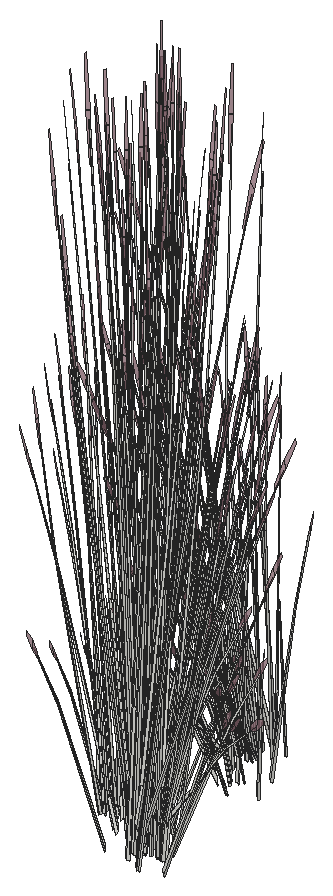
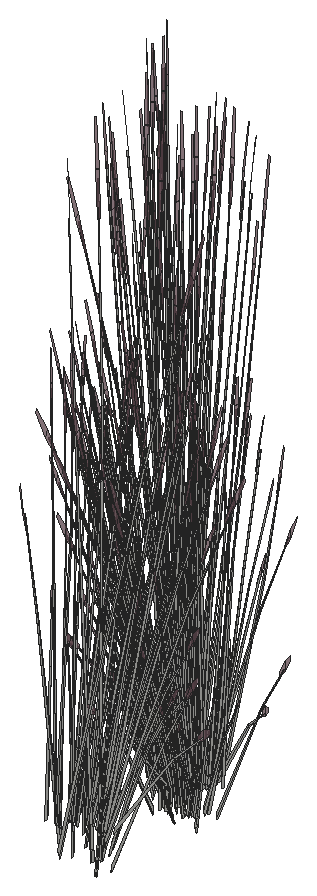
# SketchUp Ruby script. Lengths in inches.
U = 1.inch
M = Sketchup.active_model
def pt(a) = Geom::Point3d.new(a.map { |v| v * U })
def face(e, loops, mat)
  f = e.add_face(loops[0].map { |a| pt(a) })
  loops[1..].each { |l| e.add_face(l.map { |a| pt(a) }).erase! }
  f.material = f.back_material = mat if mat
  f
end
# faces: each face lists its corners as indices into pts; further lists are holes
def faces(e, pts, list, mat = nil) = list.each { |f| face(e, (f[0].is_a?(Array) ? f : [f]).map { |l| l.map { |i| pts[i] } }, mat) }
# xy, xz, yz: faces in a plane at the given z, y or x. An outline is a flat list of corners, or four numbers for a rectangle; further outlines are holes
def ring(l) = l.size == 4 ? [[l[0], l[1]], [l[2], l[1]], [l[2], l[3]], [l[0], l[3]]] : l.each_slice(2).to_a
def flat(e, list, mat, &to3) = list.each { |f| face(e, (f[0].is_a?(Array) ? f : [f]).map { |l| ring(l).map { |u, v| to3.(u, v) } }, mat) }
def xy(e, z, list, mat = nil) = flat(e, list, mat) { |x, y| [x, y, z] }
def xz(e, y, list, mat = nil) = flat(e, list, mat) { |x, z| [x, y, z] }
def yz(e, x, list, mat = nil) = flat(e, list, mat) { |y, z| [x, y, z] }
def lines(e, pts, list) = list.each { |a, b| e.add_line(pt(pts[a]), pt(pts[b])) }
# prism: a flat outline (further loops are holes) pulled along v
def prism(e, loops, v, mat = nil)
  f = face(e, loops, mat); d = Geom::Vector3d.new(v.map { |x| x * U })
  f.pushpull(f.normal.samedirection?(d) ? d.length : -d.length)
end
def box(e, o, s, mat = nil) = prism(e, [[o, [o[0] + s[0], o[1], o[2]], [o[0] + s[0], o[1] + s[1], o[2]], [o[0], o[1] + s[1], o[2]]]], [0, 0, s[2]], mat)
def at(x, y, z, deg = 0) = Geom::Transformation.translation(pt([x, y, z])) * Geom::Transformation.rotation(ORIGIN, Z_AXIS, deg.degrees)
def axes(o, x, y, z) = Geom::Transformation.new([*x, 0, *y, 0, *z, 0, *pt(o).to_a, 1])
def part(name) = M.definitions.add(name)
# library, detail: a bought-in or finely detailed component or shape, given as its bounding box
def library(name, o, s) = part(name).tap { |d| box(d.entities, o, s) }
def detail(e, o, s) = box(e.add_group.entities, o, s)
def put(e, d, t, mat = nil) = e.add_instance(d, t).tap { |i| i.material = mat if mat }
def group(e, t, mat = nil) = e.add_group.tap { |g| g.transformation = t; g.material = mat if mat }.entities
root = M.entities
M.materials.add("LightPink_Translucent").color = [144, 107, 117]
M.materials["LightPink_Translucent"].alpha = 0.75
c1 = part("blade")
p = [[2.15,0.21,22],[0,0.17,0],[0.09,0.45,0],[2.18,0.31,22],[2.29,0.31,22],[0.38,0.45,0],
  [2.48,0.24,33],[2.49,0.24,33],[2.48,0.22,33]]
faces(c1.entities,p,[[0,1,2,3],[4,5,2,3],[6,3,4,7],[8,0,3,6]])
c2 = part("seeds")
p = [[0.3,-0.1,1.38],[-0.01,-0.03,1.59],[-0.01,-0.03,0.03],[0.14,-0.07,-0.07],[0.29,-0.03,3],[0.15,0.01,3.11]]
faces(c2.entities,p,[[0,1,2,3],[1,0,4,5]],"LightPink_Translucent")
c3 = part("blade with seeds")
put(c3.entities,c1,at(0,0,0))
put(c3.entities,c2,axes([2.4,0.25,30.99],[1.5799,-0.05474,1.17369],[-0.12525,1.92788,0.29478],[-0.07173,-0.02425,1.56792]))
put(root,c3,axes([416.83,611.77,155.49],[0.51796,0.09937,0.38653],[-0.10541,0.56124,0.15168],[-0.07569,-0.05419,1.34202]))
put(root,c3,axes([419.57,611.36,154.75],[-0.02142,-0.07161,1.48974],[0.14855,-0.41887,-0.22758],[0.14984,-0.00603,0.25375]))
put(root,c3,axes([415.14,611.29,154.75],[0.01039,0.07433,1.48974],[-0.20952,0.38819,-0.22758],[-0.14882,-0.01957,0.25375]))
put(root,c3,axes([417.33,610.88,155.79],[-0.24618,-0.39589,0.37796],[0.37289,-0.27878,-0.1819],[0.07967,0.04899,1.2135]))
put(root,c3,axes([416.0625,612.6875,155.21],[-0.09626,-0.41098,-0.2617],[0.38233,-0.1167,0.2617],[-0.07708,-0.04739,1.17405]))
put(root,c3,axes([416.55,612.66,155.58],[0.44036,-0.12519,0.14904],[0.10874,0.46588,0.29641],[-0.03927,-0.06788,1.35512]))
put(root,c3,axes([417.46,610.9,155.75],[0.41376,-0.31314,-0.2458],[0.27514,0.44246,-0.42242],[0.10209,0.04493,1.34921]))
put(root,c3,axes([419.1,611.73,157.32],[0.34057,0.13158,-0.29918],[-0.09933,0.38387,0.38624],[0.13712,-0.0352,0.73904]))
put(root,c3,axes([415.96,612.86,155.2],[-0.38354,-0.23583,-0.41945],[0.22925,-0.42288,0],[-0.08735,-0.05371,1.33059]))
put(root,c3,axes([418.5,610.07,155.2],[0.38354,0.23583,-0.41945],[-0.22925,0.42288,0],[0.08735,0.05371,1.33059]))
put(root,c3,axes([415.1,611.12,157.32],[-0.34057,-0.13158,-0.29918],[0.09933,-0.38387,0.38624],[-0.13712,0.0352,0.73904]))
put(root,c3,axes([417.78,611.42,155.36],[0.45849,0,0],[0,0.4883,0],[0,0,1.50718]))
put(root,c3,axes([417,612.03,155.75],[-0.41376,0.31314,-0.2458],[-0.27514,-0.44246,-0.42242],[-0.10209,-0.04493,1.34921]))
put(root,c3,axes([417.91,610.27,155.58],[-0.44036,0.12519,0.14904],[-0.10874,-0.46588,0.29641],[0.03927,0.06788,1.35512]))
put(root,c3,axes([418.18,611.25,156.77],[-0.16998,0.01068,1.44779],[0.11276,-0.46299,0.11706],[0.24224,0.02864,0.61892]))
put(root,c3,axes([418.4,610.25,155.21],[0.09626,0.41098,-0.2617],[-0.38233,0.1167,0.2617],[0.07708,0.04739,1.17405]))
put(root,c3,axes([419.05,611.89,157.49],[0.15051,0.3216,0.05432],[-0.27447,0.15741,0.42765],[0.12099,-0.03106,0.65209]))
put(root,c3,axes([417.63,611.17,155.5],[-0.51796,-0.09937,0.41563],[0.10541,-0.56124,0.1631],[0.07569,0.05419,1.44303]))
put(root,c3,axes([419.03,611.78,157.49],[-0.11578,0.43006,0.40553],[-0.38064,-0.14706,0.33437],[0.14969,-0.02584,0.83914]))
put(root,c3,axes([417.21,612.55,155.36],[-0.13371,-0.40664,0],[0.38182,-0.1424,0],[0,0,1.30413]))
put(root,c3,axes([416.96,612.17,155.7],[-0.07906,0.42093,0.12232],[-0.38625,-0.07307,-0.3493],[-0.07029,-0.04322,1.07074]))
put(root,c3,axes([415.46,611.08,157.76],[0.34057,0.13158,0.29918],[-0.09933,0.38387,-0.38624],[-0.13712,0.0352,0.73904]))
put(root,c3,axes([417.71,612.5,155.34],[0.43024,-0.16003,-0.16218],[0.15118,0.46099,0.00007],[0.04749,-0.01769,1.46908]))
put(root,c3,axes([417.86,612.69,155.58],[0.11838,-0.46875,0.14904],[0.43321,0.13265,0.29641],[-0.07483,0.00228,1.35512]))
put(root,c3,axes([417.77,611.625,155.36],[0.28606,0.30466,0],[-0.28606,0.30466,0],[0,0,1.42996]))
put(root,c3,axes([416.14,611.05,156.32],[0.11649,-0.06823,1.49584],[0.04017,0.47639,0.11706],[-0.25231,0.06321,0.53462]))
put(root,c3,axes([418.54,611.49,155.58],[-0.32198,-0.34356,0.14904],[0.32447,-0.33323,0.29641],[-0.03556,0.07016,1.35512]))
put(root,c3,axes([419.83,611.81,155.83],[-0.2532,0.07787,0.97034],[0.11918,-0.32181,0.71294],[0.13432,0.02202,0.21373]))
put(root,c3,axes([417.12,612.74,155.35],[-0.41314,-0.21175,0],[0.19883,-0.43999,0],[0,0,1.37455]))
put(root,c3,axes([417.46,612.17,155.58],[-0.40016,-0.37963,-0.21282],[0.33672,-0.42629,0.46574],[-0.10776,0.04441,1.42109]))
put(root,c3,axes([416.41,612.9,155.59],[0.38354,0.23583,0.41945],[-0.22925,0.42288,0],[-0.08735,-0.05371,1.33059]))
put(root,c3,axes([417.76,611.27,155.79],[0.19883,-0.425,0.37796],[0.41314,0.20454,-0.1819],[0,0.09797,1.2135]))
put(root,c3,axes([419.71,613.17,157.47],[-0.03706,-0.04129,1.49853],[0.08106,-0.44261,-0.1416],[0.14596,-0.02828,0.26519]))
put(root,c3,axes([414.89,611.375,157.48],[-0.06692,0.06124,1.47793],[0.00569,0.44742,-0.23373],[-0.15339,0.05818,0.11853]))
put(root,c3,axes([417.68,611.51,155.43],[0,0.54548,-0.04762],[-0.51243,0,0],[0,0.01714,1.5153]))
put(root,c3,axes([415.34,611.3125,157.45],[-0.11102,0.42903,-0.43168],[-0.38064,-0.14706,-0.33437],[-0.15325,0.03934,0.82598]))
put(root,c3,axes([415.32,610.95,157.75],[0.20619,0.42709,-0.10273],[-0.36595,0.20988,-0.57019],[-0.15422,0.05635,0.8664]))
put(root,c3,axes([417.72,611.125,155.36],[0.24618,0.39589,-0.37796],[-0.37289,0.27878,0.1819],[0.07967,0.04899,1.2135]))
put(root,c3,axes([419.39,612.8,156.8125],[-0.07843,-0.39649,-0.0295],[0.37072,-0.09115,-0.13375],[0.07742,0.02514,0.44114]))
put(root,c3,axes([416.1875,613.15,155.5],[-0.25622,0.47263,0],[-0.42866,-0.26357,-0.43598],[-0.09763,-0.06003,1.38303]))
put(root,c3,axes([418.43,612.79,157.75],[0.02194,-0.47967,-0.10273],[0.41546,0.01311,-0.57019],[0.16001,0.03332,0.8664]))
put(root,c3,axes([418.8,611.51,155.59],[0,-0.47166,0.41945],[0.45849,0,0],[0,0.10742,1.33059]))
put(root,c3,axes([417.66,611.86,155.79],[0.44501,-0.02912,0.37796],[0.04024,0.48332,-0.1819],[-0.07967,0.04899,1.2135]))
put(root,c3,axes([417.93,611.37,155.7],[0.38182,-0.13755,0.12232],[0.13371,0.39278,-0.3493],[0,0.08644,1.07074]))
put(root,c3,axes([418.36,612.6,157.76],[-0.23317,-0.29531,0.29918],[0.26625,-0.27955,-0.38624],[0.13527,0.04253,0.73904]))
put(root,c3,axes([417.26,612.09,155.36],[-0.44501,0.02912,-0.37796],[-0.04024,-0.48332,0.1819],[-0.07967,0.04899,1.2135]))
put(root,c3,axes([419.35,612.32,155.68],[-0.0987,-0.116,1.20808],[0.12841,-0.38374,-0.25981],[0.19968,0.05198,0.51652]))
put(root,c3,axes([417.59,612.75,155.36],[0.41314,0.21175,0],[-0.19883,0.43999,0],[0,0,1.47801]))
put(root,c3,axes([418.79,612.5,157.48],[0.08791,-0.00798,1.47793],[0.24113,-0.36643,-0.23373],[0.15637,0.04837,0.11853]))
put(root,c3,axes([417.75,613.21,155.35],[-0.25302,-0.47428,-0.04344],[0.42866,-0.26357,0.43598],[-0.10563,0.04516,1.38235]))
put(root,c3,axes([417.66,612.07,155.7],[0.30276,0.28338,0.12232],[-0.25254,0.31972,-0.3493],[-0.07029,0.04322,1.07074]))
put(root,c3,axes([415.27,612.14,157.49],[-0.10163,-0.43409,0.40553],[0.39868,-0.07534,0.33437],[-0.1175,0.10209,0.83914]))
put(root,c3,axes([415.19,612.06,157.49],[-0.28133,-0.19836,0.05432],[0.16379,-0.28248,0.42765],[-0.0902,0.09132,0.65209]))
put(root,c3,axes([415.32,611.54,156.77],[0.14219,-0.09977,1.44779],[0.11971,0.461,0.11706],[-0.22323,0.10419,0.61892]))
put(root,c3,axes([418.45,612.56,157.7],[0.40965,0.01136,-0.60019],[-0.02751,0.47821,0.07243],[0.17355,0.05047,0.84903]))
put(root,c3,axes([417.99,612.94,155.59],[0.38354,-0.23583,0.41945],[0.22925,0.42288,0],[-0.08735,0.05371,1.33059]))
put(root,c3,axes([417.44,612.57,155.43],[0.17817,0.54185,-0.05079],[-0.50909,0.18987,0],[0.00622,0.01892,1.45452]))
put(root,c3,axes([417.64,613.15,155.21],[-0.38233,-0.1167,-0.2617],[0.09626,-0.41098,0.2617],[-0.07708,0.04739,1.17405]))
put(root,c3,axes([414.88,612.32,155.68],[0.14242,0.03872,1.20808],[0.09179,0.39548,-0.25981],[-0.19345,0.07403,0.51652]))
put(root,c3,axes([415.52,612,157.76],[0.35672,-0.06741,0.29918],[0.09419,0.38534,-0.38624],[-0.10222,0.1035,0.73904]))
put(root,c3,axes([419.12,611.59,155.5],[0.51243,0,0],[0,0.52715,-0.43598],[0,0.12006,1.38303]))
put(root,c3,axes([414.14,611.83,157.47],[0.0523,0.01265,1.49853],[0.16179,0.41674,-0.1416],[-0.10706,0.10938,0.26519]))
put(root,c3,axes([418.91,611.86,155.35],[-0.51218,-0.00377,-0.04204],[0,-0.52715,0.42192],[-0.0161,0.12,1.33776]))
put(root,c3,axes([417.8,611.4,155.75],[0.46151,0.22505,-0.2458],[-0.22222,0.475,-0.42242],[0.0145,0.11662,1.34921]))
put(root,c3,axes([414.58,613.15,155.83],[0.17079,-0.21377,0.97034],[0.06739,0.33841,0.71294],[-0.12342,0.0606,0.21373]))
put(root,c3,axes([418.69,612.75,157.32],[0.23317,0.29531,-0.29918],[-0.26625,0.27955,0.38624],[0.13527,0.04253,0.73904]))
put(root,c3,axes([418.8,611.93,155.21],[-0.28606,0.29428,-0.2617],[-0.28606,-0.29428,0.2617],[0,0.09479,1.17405]))
put(root,c3,axes([417.57,611.96,155.75],[0.04775,0.53819,-0.2458],[-0.49736,0.03254,-0.42242],[-0.08758,0.07169,1.34921]))
put(root,c3,axes([418.57,612.87,157.49],[-0.02064,0.35866,0.05432],[-0.3116,-0.00983,0.42765],[0.11936,0.03753,0.65209]))
put(root,c3,axes([417.75,611.75,155.36],[-0.19883,0.425,-0.37796],[-0.41314,-0.20454,0.1819],[0,0.09797,1.2135]))
put(root,c3,axes([415.23,612.23,157.32],[-0.35672,0.06741,-0.29918],[-0.09419,-0.38534,0.38624],[-0.10222,0.1035,0.73904]))
put(root,c3,axes([418.6,612.75,157.49],[-0.30217,0.31079,0.40553],[-0.2606,-0.33005,0.33437],[0.14177,0.05733,0.83914]))
put(root,c3,axes([414.71,613.09,158.26],[0.36162,0.1259,-0.05481],[-0.11124,0.3875,-0.2485],[-0.05915,0.05883,0.81966]))
put(root,c3,axes([417.64,613.11,157.76],[-0.06329,-0.37991,0.29918],[0.36182,-0.10032,-0.38624],[0.09718,0.10887,0.73904]))
put(root,c3,axes([417.76,612.97,155.46],[0.51304,0.1533,0.25983],[-0.12835,0.54797,-0.30828],[-0.08491,0.06858,1.39295]))
put(root,c3,axes([417.73,613.34,155.2],[-0.38354,0.23583,-0.41945],[-0.22925,-0.42288,0],[-0.08735,0.05371,1.33059]))
put(root,c3,axes([419,611.95,155.2],[0,0.47166,-0.41945],[-0.45849,0,0],[0,0.10742,1.33059]))
put(root,c3,axes([417.86,612,156.77],[-0.15222,-0.08126,1.44779],[0.31502,-0.34091,0.11706],[0.19634,0.15379,0.61892]))
put(root,c3,axes([417.88,610.93,157.27],[-0.35411,-0.24507,1.16821],[0.37391,-0.38156,0.50405],[0.11425,0.22994,1.12919]))
put(root,c3,axes([415.33,611.96,157.75],[0.37908,0.26007,-0.10273],[-0.21839,0.37663,-0.57019],[-0.1071,0.13092,0.8664]))
put(root,c3,axes([418.42,612.92,155.83],[-0.23074,-0.13562,0.97034],[0.29794,-0.1378,0.71294],[0.08036,0.11673,0.21373]))
put(root,c3,axes([417.61,613.31,157.75],[0.2442,-0.40372,-0.10273],[0.35364,0.23259,-0.57019],[0.12293,0.11406,0.8664]))
put(root,c3,axes([415.84,611.85,156.77],[0.10236,-0.14492,1.44779],[0.25844,0.39118,0.11706],[-0.17726,0.17814,0.61892]))
put(root,c3,axes([415.52,612.27,157.45],[0.10528,0.43067,-0.43168],[-0.39868,0.07534,-0.33437],[-0.11425,0.11568,0.82598]))
put(root,c3,axes([416,612.77,157.76],[0.27728,-0.24833,0.29918],[0.26248,0.28355,-0.38624],[-0.03994,0.14407,0.73904]))
put(root,c3,axes([418.08,613.27,155.5],[0.25622,0.47263,0],[-0.42866,0.26357,-0.43598],[-0.09763,0.06003,1.38303]))
put(root,c3,axes([417.29,613.65,157.47],[0.00121,-0.0571,1.49853],[0.35119,-0.25193,-0.1416],[0.12199,0.08992,0.26519]))
put(root,c3,axes([418.48,613.43,154.75],[0.02986,-0.06809,1.48974],[0.37589,-0.20055,-0.22758],[0.11396,0.1038,0.25375]))
put(root,c3,axes([417.86,611.4,155.89],[-0.01119,-0.44408,1.19347],[0.50665,0.11511,0.50532],[-0.11983,0.243,1.12654]))
put(root,c3,axes([415.75,612.99,157.49],[-0.33677,-0.02198,0.05432],[0.00923,-0.33185,0.42765],[-0.03524,0.12712,0.65209]))
put(root,c3,axes([415.03,613.37,154.75],[0.05497,0.04712,1.48974],[0.09321,0.43661,-0.22758],[-0.12183,0.0931,0.25375]))
put(root,c3,axes([415.85,613.02,157.49],[-0.29182,-0.32181,0.40553],[0.3099,-0.27755,0.33437],[-0.05383,0.15098,0.83914]))
put(root,c3,axes([417.9,613.11,157.45],[0.40438,-0.11212,-0.43168],[0.07074,0.4246,-0.33437],[0.10862,0.12168,0.82598]))
put(root,c3,axes([416.78,613.17,157.76],[0.12355,-0.36271,0.29918],[0.36044,0.10579,-0.38624],[0.03305,0.14603,0.73904]))
put(root,c3,axes([418.46,613.54,155.75],[-0.26279,-0.01479,0.88755],[0.17355,-0.31417,0.49003],[0.10382,0.11162,0.6962]))
put(root,c3,axes([417.7,613.46,157.49],[-0.18625,0.29962,0.05432],[-0.26523,-0.17444,0.42765],[0.08575,0.09606,0.65209]))
put(root,c3,axes([417.26,614.47,158.26],[0.28319,-0.27058,-0.05481],[0.25948,0.29635,-0.2485],[0.01827,0.08397,0.81966]))
put(root,c3,axes([417.78,613.375,157.49],[-0.4076,0.10824,0.40553],[-0.07074,-0.4246,0.33437],[0.09586,0.12514,0.83914]))
put(root,c3,axes([415.77,612.2,156.77],[0.0763,-0.16212,1.44779],[0.3201,0.3355,0.11706],[-0.1444,0.2091,0.61892]))
put(root,c3,axes([417.6,612.78,155.68],[0.00723,-0.15635,1.20808],[0.34559,-0.17464,-0.25981],[0.10668,0.18713,0.51652]))
put(root,c3,axes([416.66,613.5,157.49],[-0.30197,0.1603,0.05432],[-0.1478,-0.29231,0.42765],[0.02916,0.12885,0.65209]))
put(root,c3,axes([415.85,613.12,157.32],[-0.27728,0.24833,-0.29918],[-0.26248,-0.28355,0.38624],[-0.03994,0.14407,0.73904]))
put(root,c3,axes([414.9,613.04,157.48],[-0.01019,0.09334,1.47793],[0.28908,0.3247,-0.23373],[-0.07568,0.15355,0.11853]))
put(root,c3,axes([415.82,612.83,158.05],[0.45039,0.02337,-0.11403],[-0.01231,0.44247,-0.63292],[-0.03129,0.17041,0.9617]))
put(root,c3,axes([416.66,613.33,157.75],[0.40102,-0.2196,-0.10273],[0.19707,0.38974,-0.57019],[0.05291,0.16424,0.8664]))
put(root,c3,axes([416.77,613.47,157.77],[-0.4038,-0.12331,0.45013],[0.13808,-0.40538,0.37115],[0.02427,0.15942,0.93144]))
put(root,c3,axes([416.03,614.08,155.83],[-0.01061,-0.28045,0.97034],[0.26501,0.20003,0.71294],[-0.05212,0.13367,0.21373]))
put(root,c3,axes([416.73,613.41,154.75],[0.06632,-0.02567,1.48974],[0.39894,0.14126,-0.22758],[0.01167,0.15921,0.25375]))
put(root,c3,axes([416.13,613,157.72],[0.29336,0.31691,-0.47917],[-0.3099,0.27755,-0.37115],[-0.04464,0.16102,0.91684]))
put(root,c3,axes([415.8125,613.48,155.88],[0.37228,-0.08352,0.05498],[0.08559,0.3365,-0.7291],[-0.0236,0.17034,0.65354]))
put(root,c3,axes([417,613.31,157.45],[0.40284,0.11824,-0.43168],[-0.13808,0.40538,-0.33437],[0.03694,0.16321,0.82598]))
put(root,c3,axes([417.23,612.47,156.77],[-0.09368,-0.15143,1.44779],[0.43286,-0.12749,0.11706],[0.09783,0.23774,0.61892]))
put(root,c3,axes([416.82,613.56,157.32],[-0.12355,0.36271,-0.29918],[-0.36044,-0.10579,0.38624],[0.03305,0.14603,0.73904]))
put(root,c3,axes([416.04,612.86,158],[-0.01066,0.43628,-0.66621],[-0.44902,-0.0293,0.0804],[-0.04739,0.18483,0.94242]))
put(root,c3,axes([414.87,614,157.47],[0.04649,-0.02848,1.49853],[0.38427,0.18941,-0.1416],[-0.00903,0.15771,0.26519]))
put(root,c3,axes([416.46,612.55,156.77],[-0.01003,-0.18103,1.44779],[0.43473,0.12009,0.11706],[-0.02689,0.25798,0.61892]))
put(root,c3,axes([416.85,613.23,157.7],[0.19559,0.38351,-0.60019],[-0.40262,0.21373,0.07243],[0.04574,0.1853,0.84903]))
put(root,c3,axes([416.2,621.26,157.125],[0.09368,0.15143,1.44779],[-0.43286,0.12749,0.11706],[-0.09783,-0.23774,0.61892]))
put(root,c3,axes([415.72,613.83,155.68],[0.12932,-0.07441,1.20808],[0.31929,0.22435,-0.25981],[-0.09503,0.19413,0.51652]))
put(root,c3,axes([416.91,620.25,157.83],[-0.06268,-0.06613,1.47793],[-0.4183,0.04193,-0.23373],[-0.06676,-0.15817,0.11853]))
put(root,c3,axes([416.5625,614.2,157.48],[0.05195,0.07595,1.47793],[0.41921,0.02984,-0.23373],[0.04216,0.1675,0.11853]))
put(root,c3,axes([417.88,621.04,156.04],[-0.11649,0.09547,1.20808],[-0.34886,-0.1671,-0.25981],[0.06467,-0.20781,0.51652]))
put(root,c3,axes([417.35,621.37,158.06],[-0.19559,-0.38351,-0.60019],[0.40262,-0.21373,0.07243],[-0.04574,-0.1853,0.84903]))
put(root,c3,axes([416.08,620.86,156.04],[-0.02482,0.15429,1.20808],[-0.36278,0.12916,-0.25981],[-0.0848,-0.19943,0.51652]))
put(root,c3,axes([417.02,620.52,155.11],[-0.06874,0.01699,1.48974],[-0.38012,-0.19128,-0.22758],[0.00638,-0.15955,0.25375]))
put(root,c3,axes([418.17,621.75,158.06],[0.01066,-0.43628,-0.60019],[0.44902,0.0293,0.07243],[0.04739,-0.18483,0.84903]))
put(root,c3,axes([415.89,613.47,156.33],[0.009,-0.24349,1.30391],[0.40497,0.12861,0.18019],[-0.03509,0.2595,0.61571]))
put(root,c3,axes([418.79,621.07,157.83],[-0.00396,-0.09387,1.47793],[-0.33411,-0.2713,-0.23373],[0.05166,-0.16446,0.11853]))
put(root,c3,axes([417.39,621.05,157.68],[0.12355,-0.36271,-0.29918],[0.36044,0.10579,0.38624],[-0.03305,-0.14603,0.73904]))
put(root,c3,axes([417.66,621.53,157.125],[-0.0763,0.16212,1.44779],[-0.3201,-0.3355,0.11706],[0.1444,-0.2091,0.61892]))
put(root,c3,axes([418.7,620.73,157.83],[-0.04162,0.03603,1.49853],[-0.40776,-0.12155,-0.1416],[-0.01476,-0.15722,0.26519]))
put(root,c3,axes([417.21,621.29,157.81],[-0.40284,-0.11824,-0.43168],[0.13808,-0.40538,-0.33437],[-0.03694,-0.16321,0.82598]))
put(root,c3,axes([417.46,620.28,156.1875],[0.05257,0.27504,0.97034],[-0.29163,-0.15233,0.71294],[0.03138,-0.14083,0.21373]))
put(root,c3,axes([418.08,621.6,157.81],[-0.29336,-0.31691,-0.43168],[0.3099,-0.27755,-0.33437],[0.04464,-0.16102,0.82598]))
put(root,c3,axes([416.49,620.04,157.83],[-0.00765,0.05653,1.49853],[-0.37706,0.20517,-0.1416],[-0.11096,-0.10488,0.26519]))
put(root,c3,axes([416.4,621.04,158.15],[0.45651,-0.12123,0.45419],[0.07923,0.47555,0.3745],[-0.10736,-0.14016,0.93983]))
put(root,c3,axes([417.43,621.13,157.85],[0.4038,0.12331,0.40553],[-0.13808,0.40538,0.33437],[-0.02427,-0.15942,0.83914]))
put(root,c3,axes([417.55,621.27,158.1],[-0.40102,0.2196,-0.10273],[-0.19707,-0.38974,-0.57019],[-0.05291,-0.16424,0.8664]))
put(root,c3,axes([418.38,621.77,158.1],[-0.45039,-0.02337,-0.10273],[0.01231,-0.44247,-0.57019],[0.03129,-0.17041,0.8664]))
put(root,c3,axes([418.35,621.48,157.68],[0.27728,-0.24833,-0.29918],[0.26248,0.28355,0.38624],[0.03994,-0.14407,0.73904]))
put(root,c3,axes([415.96,620.61,156.1875],[0.21377,0.16416,0.97034],[-0.31132,0.09868,0.71294],[-0.06661,-0.12616,0.21373]))
put(root,c3,axes([417.54,621.1,157.85],[0.30197,-0.1603,0.05432],[0.1478,0.29231,0.42765],[-0.02916,-0.12885,0.65209]))
put(root,c3,axes([416.47,621.48,158.06],[-0.34944,-0.22798,-0.60019],[0.24834,-0.39949,0.07243],[-0.1266,-0.13612,0.84903]))
put(root,c3,axes([416.35,621.18,157.68],[-0.06329,-0.37991,-0.29918],[0.36182,-0.10032,0.38624],[-0.09718,-0.10887,0.73904]))
put(root,c3,axes([416.51,621.14,157.85],[0.18625,-0.29962,0.05432],[0.26523,0.17444,0.42765],[-0.08575,-0.09606,0.65209]))
put(root,c3,axes([415.79,621.1,155.11],[-0.0397,0.06213,1.48974],[-0.40116,0.13396,-0.22758],[-0.09691,-0.12186,0.25375]))
put(root,c3,axes([415.57,621.73,157.125],[0.15222,0.08126,1.44779],[-0.31502,0.34091,0.11706],[-0.19634,-0.15379,0.61892]))
put(root,c3,axes([418.7,621.33,155.11],[-0.06134,-0.03716,1.48974],[-0.15755,-0.41512,-0.22758],[0.10629,-0.11265,0.25375]))
put(root,c3,axes([417.43,621.43,158.12],[-0.12355,0.36271,0.29918],[-0.36044,-0.10579,-0.38624],[-0.03305,-0.14603,0.73904]))
put(root,c3,axes([416.31,621.49,157.81],[-0.40438,0.11212,-0.43168],[-0.07074,-0.4246,-0.33437],[-0.10862,-0.12168,0.82598]))
put(root,c3,axes([418.35,621.58,157.85],[0.29182,0.32181,0.40553],[-0.3099,0.27755,0.33437],[0.05383,-0.15098,0.83914]))
put(root,c3,axes([416.59,621.11,158.4375],[-0.2735,0.45217,-0.11506],[-0.39608,-0.2605,-0.63862],[-0.13768,-0.12775,0.97037]))
put(root,c3,axes([418.46,621.61,157.85],[0.33677,0.02198,0.05432],[-0.00923,0.33185,0.42765],[0.03524,-0.12712,0.65209]))
put(root,c3,axes([418.21,621.84,158.12],[-0.27728,0.24833,0.29918],[-0.26248,-0.28355,-0.38624],[0.03994,-0.14407,0.73904]))
put(root,c3,axes([418.7,622.5,158.06],[0.21406,-0.37215,-0.60019],[0.37511,0.26448,0.07243],[0.12781,-0.13483,0.84903]))
put(root,c3,axes([416.38,621.42,155.86],[-0.25622,-0.47263,0],[0.42866,-0.26357,-0.43598],[0.09763,-0.06003,1.38303]))
put(root,c3,axes([418.6875,622.33,157.81],[-0.10528,-0.43067,-0.43168],[0.39868,-0.07534,-0.33437],[0.11425,-0.11568,0.82598]))
put(root,c3,axes([416.95,620.85,155.65],[-0.28319,0.27058,-0.03288],[-0.25948,-0.29635,-0.1491],[-0.01827,-0.08397,0.4918]))
put(root,c3,axes([415.54,620.98,157.83],[-0.08817,-0.00333,1.47793],[-0.28072,0.33293,-0.23373],[-0.14978,-0.06803,0.11853]))
put(root,c3,axes([418.875,622.64,158.1],[-0.37908,-0.26007,-0.10273],[0.21839,-0.37663,-0.57019],[0.1071,-0.13092,0.8664]))
put(root,c3,axes([417.31,624.06,156.66],[0.35414,0.19019,1.27785],[-0.34693,0.40974,0.50532],[-0.1554,-0.24285,1.07126]))
put(root,c3,axes([416.56,621.49,158.12],[0.06329,0.37991,0.29918],[-0.36182,0.10032,-0.38624],[-0.09718,-0.10887,0.73904]))
put(root,c3,axes([415.46,622.74,155.56],[0,-0.47166,-0.41945],[0.45849,0,0],[0,-0.10742,1.33059]))
put(root,c3,axes([416.73,621.35,155.56],[0.38354,-0.23583,-0.41945],[0.22925,0.42288,0],[0.08735,-0.05371,1.33059]))
put(root,c3,axes([419.01,622.16,156.04],[-0.1464,-0.01397,1.20808],[-0.14998,-0.37477,-0.25981],[0.17985,-0.10602,0.51652]))
put(root,c3,axes([415.48,621.74,158.15],[0.33843,-0.34808,0.45419],[0.29188,0.36965,0.3745],[-0.15878,-0.06421,0.93983]))
put(root,c3,axes([419.81,622.53,157.83],[-0.05353,-0.00358,1.49853],[-0.22227,-0.38383,-0.1416],[0.08926,-0.1262,0.26519]))
